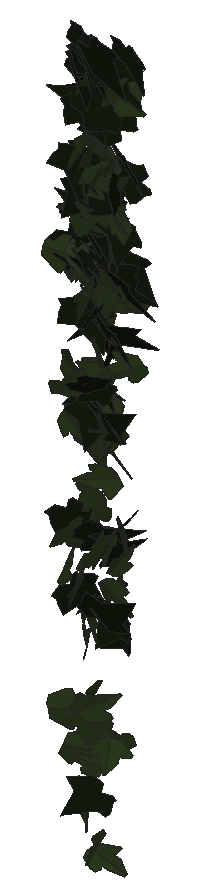
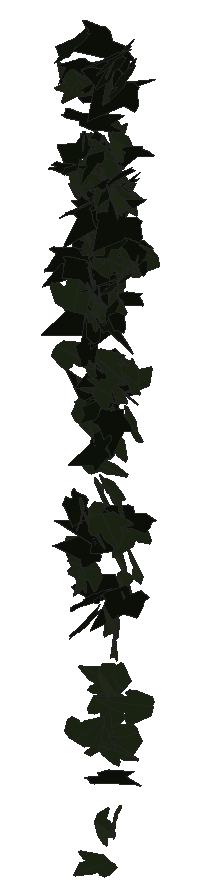
# SketchUp Ruby script. Lengths in inches.
U = 1.inch
M = Sketchup.active_model
def pt(a) = Geom::Point3d.new(a.map { |v| v * U })
def face(e, loops, mat)
  f = e.add_face(loops[0].map { |a| pt(a) })
  loops[1..].each { |l| e.add_face(l.map { |a| pt(a) }).erase! }
  f.material = f.back_material = mat if mat
  f
end
# faces: each face lists its corners as indices into pts; further lists are holes
def faces(e, pts, list, mat = nil) = list.each { |f| face(e, (f[0].is_a?(Array) ? f : [f]).map { |l| l.map { |i| pts[i] } }, mat) }
# xy, xz, yz: faces in a plane at the given z, y or x. An outline is a flat list of corners, or four numbers for a rectangle; further outlines are holes
def ring(l) = l.size == 4 ? [[l[0], l[1]], [l[2], l[1]], [l[2], l[3]], [l[0], l[3]]] : l.each_slice(2).to_a
def flat(e, list, mat, &to3) = list.each { |f| face(e, (f[0].is_a?(Array) ? f : [f]).map { |l| ring(l).map { |u, v| to3.(u, v) } }, mat) }
def xy(e, z, list, mat = nil) = flat(e, list, mat) { |x, y| [x, y, z] }
def xz(e, y, list, mat = nil) = flat(e, list, mat) { |x, z| [x, y, z] }
def yz(e, x, list, mat = nil) = flat(e, list, mat) { |y, z| [x, y, z] }
def lines(e, pts, list) = list.each { |a, b| e.add_line(pt(pts[a]), pt(pts[b])) }
# prism: a flat outline (further loops are holes) pulled along v
def prism(e, loops, v, mat = nil)
  f = face(e, loops, mat); d = Geom::Vector3d.new(v.map { |x| x * U })
  f.pushpull(f.normal.samedirection?(d) ? d.length : -d.length)
end
def box(e, o, s, mat = nil) = prism(e, [[o, [o[0] + s[0], o[1], o[2]], [o[0] + s[0], o[1] + s[1], o[2]], [o[0], o[1] + s[1], o[2]]]], [0, 0, s[2]], mat)
def at(x, y, z, deg = 0) = Geom::Transformation.translation(pt([x, y, z])) * Geom::Transformation.rotation(ORIGIN, Z_AXIS, deg.degrees)
def axes(o, x, y, z) = Geom::Transformation.new([*x, 0, *y, 0, *z, 0, *pt(o).to_a, 1])
def part(name) = M.definitions.add(name)
# library, detail: a bought-in or finely detailed component or shape, given as its bounding box
def library(name, o, s) = part(name).tap { |d| box(d.entities, o, s) }
def detail(e, o, s) = box(e.add_group.entities, o, s)
def put(e, d, t, mat = nil) = e.add_instance(d, t).tap { |i| i.material = mat if mat }
def group(e, t, mat = nil) = e.add_group.tap { |g| g.transformation = t; g.material = mat if mat }.entities
root = M.entities
M.materials.add("1026 AP 7946 SUNNY SIDE UP").color = [254, 231, 186]
M.materials.add("efeu1").color = [18, 25, 13]
M.materials.add("efeu2").color = [43, 57, 29]
c1 = part("ivyleaf_9")
p = [[1.54,2.16,1.25],[1.36,2.04,1.19],[-0.21,0.99,0.68],[-0.71,1.11,0.82],[-0.85,0.86,0.67],[-0.8,0.17,0.21],
  [-0.9,-0.01,0.1],[-0.67,-0.16,-0.02],[-0.08,-0.08,-0.05],[-0.03,-0.6,-0.4],[0.65,-0.88,-0.66],[0.83,-0.6,-0.49],
  [1.29,-0.42,-0.43],[1.8125,-0.07,-0.26],[1.21,0.44,0.15]]
faces(c1.entities,p,[[0,1,2,3,4,5,6,7,8,9,10,11,12,13,14]],"efeu1")
c2 = part("ivyleaf_10")
p = [[0,0.5,-0.03],[-0.0625,2.02,-0.43],[-0.19,2.01,-0.46],[-0.54,1.05,-0.29],[-0.52,0.625,-0.18],[-0.83,0.76,-0.28],
  [-1.16,0.64,-0.33],[-1.15,0.33,-0.24],[-0.77,-0.39,0.02],[-0.3,-0.51,0.16],[0.04,-0.48,0.23],[-0.02,2.01,-0.4375],
  [-0.06,2.01,-0.43],[0.04,-0.49,0.23],[0.67,-0.49,0.14],[1.38,0.36,-0.2],[1.375,0.51,-0.24],[0.81,0.65,-0.19],
  [0.62,0.59,-0.15],[0.6,1.09,-0.28],[0.5,1.23,-0.31]]
faces(c2.entities,p,[[0,1,2,3,4,5,6,7,8,9,10],[11,12,0,13,14,15,16,17,18,19,20]],"efeu2")
put(root,c1,axes([110.53,212.48,267.24],[0.21035,-0.21882,-0.03248],[-0.0439,0.01838,-0.2637],[0.34456,0.13592,-0.01377]),"1026 AP 7946 SUNNY SIDE UP")
put(root,c2,axes([110.8,212.3,263.71],[-0.32704,0.09178,0.06371],[-0.11121,-0.01038,-0.23118],[-0.13325,-0.21659,0.03658]),"1026 AP 7946 SUNNY SIDE UP")
put(root,c2,axes([110.62,212.41,263.32],[-0.07774,0.00799,0.24744],[0.17026,-0.21813,0.02917],[0.33727,0.11196,0.04231]),"1026 AP 7946 SUNNY SIDE UP")
put(root,c2,axes([110.45,212.27,261.32],[0.01134,-0.01111,0.25252],[0.35732,-0.09238,-0.01174],[0.14581,0.22723,0.00913]),"1026 AP 7946 SUNNY SIDE UP")
put(root,c2,axes([110.76,212.29,264.875],[0.02476,-0.20836,0.1301],[-0.00151,-0.12778,-0.21581],[0.38407,0.01293,-0.00924]),"1026 AP 7946 SUNNY SIDE UP")
put(root,c2,axes([110.67,211.92,257.39],[0.2249,-0.21057,0.04235],[-0.014,0.04497,0.26187],[-0.33742,-0.14221,0.01736]),"1026 AP 7946 SUNNY SIDE UP")
put(root,c1,axes([110.58,212.6,263.31],[0.00854,-0.22232,0.09994],[0.03105,-0.09757,-0.22909],[0.38094,0.01294,0.01643]),"1026 AP 7946 SUNNY SIDE UP")
put(root,c2,axes([110.8,212.7,261.2],[-0.02832,-0.12839,0.19332],[-0.04264,-0.18642,-0.13465],[0.35592,-0.03255,-0.00075]),"1026 AP 7946 SUNNY SIDE UP")
put(root,c2,axes([110.41,212.01,263.67],[-0.02831,-0.07099,-0.26298],[0.4153,-0.0198,-0.01365],[-0.0244,-0.25474,0.07273]),"1026 AP 7946 SUNNY SIDE UP")
put(root,c1,axes([110.64,212.21,257.03],[0.03332,-0.08184,-0.27604],[-0.07945,0.26272,-0.0854],[0.43261,0.05455,0.00558]),"1026 AP 7946 SUNNY SIDE UP")
put(root,c2,axes([111.01,212.47,263.63],[-0.10628,-0.027,0.24128],[-0.29259,-0.14375,-0.07319],[0.22802,-0.19705,0.01854]),"1026 AP 7946 SUNNY SIDE UP")
put(root,c1,axes([110.64,212.625,265.39],[0.00168,-0.25128,-0.02336],[0.00658,0.02126,-0.2587],[0.39646,0.00071,0.00439]),"1026 AP 7946 SUNNY SIDE UP")
put(root,c1,axes([110.66,212.32,264.46],[0.32463,0.14976,0.01796],[0.0383,-0.00541,-0.26208],[-0.2338,0.20705,-0.01799]),"1026 AP 7946 SUNNY SIDE UP")
put(root,c1,axes([110.61,212.2,263.97],[-0.00886,-0.04705,-0.2482],[0.08546,0.2345,-0.04717],[0.37599,-0.05441,0.00487]),"1026 AP 7946 SUNNY SIDE UP")
put(root,c2,axes([110.53,212.18,260.33],[0.09967,0.00276,0.24211],[0.34341,-0.0906,-0.06012],[0.13651,0.22591,-0.02554]),"1026 AP 7946 SUNNY SIDE UP")
put(root,c2,axes([110.73,211.93,261.05],[-0.18233,-0.19779,0.08114],[0.05318,0.07273,0.23651],[-0.33117,0.12057,-0.00669]),"1026 AP 7946 SUNNY SIDE UP")
put(root,c2,axes([110.76,212,258.28],[-0.17012,-0.21862,-0.16272],[0.11818,0.13762,-0.25042],[0.4061,-0.13163,0.00471]),"1026 AP 7946 SUNNY SIDE UP")
put(root,c1,axes([110.63,212.1,258.58],[-0.01613,-0.09449,-0.22982],[0.12276,0.20952,-0.09412],[0.3598,-0.07572,0.02181]),"1026 AP 7946 SUNNY SIDE UP")
put(root,c1,axes([110.66,212.55,267.66],[0.03626,-0.25281,0.10174],[0.0069,-0.10019,-0.26207],[0.42754,0.02306,-0.0044]),"1026 AP 7946 SUNNY SIDE UP")
put(root,c2,axes([110.85,212.1,257.2],[0.09037,-0.22921,0.00924],[-0.00391,-0.01121,-0.24345],[0.36075,0.05729,-0.00495]),"1026 AP 7946 SUNNY SIDE UP")
put(root,c2,axes([110.93,212.48,258.51],[-0.23687,-0.16124,0.07836],[-0.06333,-0.06745,-0.22714],[0.27371,-0.15514,0.01526]),"1026 AP 7946 SUNNY SIDE UP")
put(root,c2,axes([110.89,212.4,256.77],[0.04127,-0.23909,-0.00761],[-0.00505,0.00571,-0.24774],[0.37604,0.02631,-0.00249]),"1026 AP 7946 SUNNY SIDE UP")
put(root,c2,axes([110.9,212.41,265.03],[0.13181,-0.23124,-0.04316],[-0.03213,0.03574,-0.25308],[0.36775,0.086,-0.00664]),"1026 AP 7946 SUNNY SIDE UP")
put(root,c2,axes([110.94,212.17,252.58],[0.02923,0.02776,-0.24498],[-0.05835,0.23612,0.02677],[0.37215,0.03484,0.02344]),"1026 AP 7946 SUNNY SIDE UP")
put(root,c1,axes([110.72,212.36,267.11],[0.03723,-0.22168,0.15427],[0.01536,-0.15079,-0.23049],[0.42148,0.02508,-0.00523]),"1026 AP 7946 SUNNY SIDE UP")
put(root,c1,axes([110.75,211.9375,263.59],[0.37651,0.01521,-0.04128],[-0.06017,-0.02762,-0.24602],[-0.03063,0.24122,-0.02413]),"1026 AP 7946 SUNNY SIDE UP")
put(root,c2,axes([110.6,211.9,254.76],[0.051,-0.00885,-0.28812],[0.389,0.13236,0.02602],[0.20542,-0.24844,0.02226]),"1026 AP 7946 SUNNY SIDE UP")
put(root,c2,axes([110.96,212.17,256.04],[0.02352,-0.02907,-0.24498],[-0.05789,0.23498,-0.03063],[0.37196,0.03841,0.01073]),"1026 AP 7946 SUNNY SIDE UP")
put(root,c1,axes([110.72,212.56,263.96],[0.02096,-0.18322,0.1737],[0.0948,-0.16251,-0.18663],[0.38101,0.05051,0.03688]),"1026 AP 7946 SUNNY SIDE UP")
put(root,c1,axes([110.83,212.2,267],[0.2399,0.23699,0.10471],[0.11162,0.07331,-0.28929],[-0.38895,0.16722,-0.01844]),"1026 AP 7946 SUNNY SIDE UP")
put(root,c2,axes([110.93,212.21,267.13],[-0.026,-0.18025,-0.22286],[0.04142,0.21373,-0.18517],[0.43958,-0.0308,0.00427]),"1026 AP 7946 SUNNY SIDE UP")
put(root,c1,axes([110.97,212.28,260.51],[0.27431,0.03959,-0.16722],[-0.24451,-0.04826,-0.18432],[-0.09704,0.23351,-0.00828]),"1026 AP 7946 SUNNY SIDE UP")
put(root,c2,axes([110.89,212.21,265.83],[0.05614,-0.14651,0.20226],[0.07485,-0.19133,-0.15647],[0.37892,0.0595,0.00094]),"1026 AP 7946 SUNNY SIDE UP")
put(root,c1,axes([110.91,212.17,264.85],[-0.10484,-0.16371,0.17331],[-0.0882,-0.1597,-0.18293],[0.35949,-0.08693,0.00566]),"1026 AP 7946 SUNNY SIDE UP")
put(root,c2,axes([110.64,212.09,263.5],[0.05389,-0.03015,0.26577],[0.39459,-0.06394,-0.04239],[0.10638,0.25244,0.0226]),"1026 AP 7946 SUNNY SIDE UP")
put(root,c2,axes([110.91,212.29,256.59],[-0.23412,0.18534,-0.04858],[0.0293,-0.04676,-0.24473],[-0.29969,-0.14936,0.01403]),"1026 AP 7946 SUNNY SIDE UP")
put(root,c1,axes([110.91,212.12,265.6],[-0.19456,-0.22788,-0.06174],[0.06088,0.04563,-0.26658],[0.36494,-0.1291,0.01156]),"1026 AP 7946 SUNNY SIDE UP")
put(root,c2,axes([110.74,212.64,265.71],[-0.1503,0.03877,-0.25334],[0.30139,-0.157,-0.10308],[-0.25034,-0.21229,0.028]),"1026 AP 7946 SUNNY SIDE UP")
put(root,c2,axes([110.93,211.96,263.61],[0.16078,0.07176,-0.21553],[0.09698,0.21253,0.10718],[0.33462,-0.09607,0.0725]),"1026 AP 7946 SUNNY SIDE UP")
put(root,c2,axes([111.25,212.08,253.8],[0.04147,0.05616,0.22779],[-0.35308,-0.03113,0.03561],[0.0605,-0.22017,0.05167]),"1026 AP 7946 SUNNY SIDE UP")
put(root,c2,axes([111.03,212.4,264.85],[-0.05861,-0.22767,0.10131],[0.0141,-0.10192,-0.23706],[0.39052,-0.03049,0.02377]),"1026 AP 7946 SUNNY SIDE UP")
put(root,c1,axes([110.79,212.46,267.34],[0.13987,-0.23061,0.09352],[0.03504,-0.09001,-0.25491],[0.38887,0.09105,-0.01067]),"1026 AP 7946 SUNNY SIDE UP")
put(root,c2,axes([110.84,211.93,254.1],[-0.07548,-0.05933,-0.2541],[0.28105,0.16975,-0.07701],[0.28234,-0.18483,0.00873]),"1026 AP 7946 SUNNY SIDE UP")
put(root,c2,axes([111.08,212.19,259.03],[0.28022,-0.15063,-0.09153],[-0.09917,0.06164,-0.23995],[0.25575,0.18895,0.00724]),"1026 AP 7946 SUNNY SIDE UP")
put(root,c1,axes([111.29,212.28,264.36],[-0.00489,0.05439,0.26295],[-0.40867,0.01897,-0.00733],[-0.03154,-0.25425,0.05414]),"1026 AP 7946 SUNNY SIDE UP")
put(root,c2,axes([111.0625,212.53,262.7],[-0.27687,0.14506,0.01845],[-0.05315,-0.01444,-0.23271],[-0.22343,-0.17632,0.0325]),"1026 AP 7946 SUNNY SIDE UP")
put(root,c1,axes([110.91,212.09,266.74],[0.07886,-0.22501,-0.16973],[-0.0777,0.15626,-0.23627],[0.43037,0.06944,-0.01156]),"1026 AP 7946 SUNNY SIDE UP")
put(root,c2,axes([110.97,212.28,260.03],[-0.37486,0.07125,-0.0784],[0.10308,-0.04651,-0.25534],[-0.12806,-0.24602,0.02395]),"1026 AP 7946 SUNNY SIDE UP")
put(root,c1,axes([110.97,212.53,267.52],[-0.12095,-0.23603,0.08358],[0.00689,-0.08754,-0.25442],[0.39308,-0.07109,0.03018]),"1026 AP 7946 SUNNY SIDE UP")
put(root,c2,axes([111.15,211.96,264.66],[-0.36302,-0.0868,0.06198],[-0.07017,-0.05219,-0.25222],[0.151,-0.23293,0.0318]),"1026 AP 7946 SUNNY SIDE UP")
put(root,c2,axes([111.09,212.01,265.22],[-0.08644,0.22852,0.07859],[-0.09972,0.06042,-0.23724],[-0.36479,-0.07067,0.04623]),"1026 AP 7946 SUNNY SIDE UP")
put(root,c1,axes([111.22,212.34,262.5],[-0.29277,0.18233,-0.08805],[0.07029,-0.07752,-0.26788],[-0.30944,-0.19011,0.02246]),"1026 AP 7946 SUNNY SIDE UP")
put(root,c1,axes([111.14,212.29,264.59],[-0.11265,0.14703,-0.19017],[0.10266,-0.17395,-0.16909],[-0.35767,-0.09624,0.01137]),"1026 AP 7946 SUNNY SIDE UP")
put(root,c2,axes([111.08,212.38,262.87],[0.09055,-0.22927,-0.05622],[0.00382,0.05542,-0.24269],[0.3701,0.05553,0.01626]),"1026 AP 7946 SUNNY SIDE UP")
put(root,c2,axes([111,212.4,263.13],[-0.10245,0.14727,-0.1753],[0.04335,-0.17145,-0.16395],[-0.35219,-0.06394,0.03081]),"1026 AP 7946 SUNNY SIDE UP")
put(root,c2,axes([111.03,212.0625,257.72],[0.17985,-0.19284,0.11996],[0.07845,-0.10692,-0.23136],[0.34633,0.12436,-0.00989]),"1026 AP 7946 SUNNY SIDE UP")
put(root,c1,axes([110.88,212.46,262.58],[0.09867,-0.17785,0.15419],[0.06564,-0.14494,-0.19501],[0.3606,0.07505,-0.00669]),"1026 AP 7946 SUNNY SIDE UP")
put(root,c1,axes([110.93,212.43,264.23],[0.09703,-0.23496,0.00497],[-0.00575,-0.00732,-0.25025],[0.36954,0.06158,-0.0052]),"1026 AP 7946 SUNNY SIDE UP")
put(root,c2,axes([111.26,212.24,261.44],[-0.19776,-0.11935,0.17048],[-0.1582,-0.13375,-0.1782],[0.28009,-0.15981,0.01972]),"1026 AP 7946 SUNNY SIDE UP")
put(root,c2,axes([111.13,212.1,263.07],[0.04487,-0.27898,0.06106],[0.01215,-0.06038,-0.28925],[0.44882,0.02952,0.00173]),"1026 AP 7946 SUNNY SIDE UP")
put(root,c1,axes([111.07,212.48,265.8125],[0.28706,-0.07966,-0.16819],[-0.23347,0.0668,-0.2048],[0.16345,0.23531,0.00284]),"1026 AP 7946 SUNNY SIDE UP")
put(root,c1,axes([111.125,212.49,263.02],[-0.19791,-0.18572,0.09633],[-0.03684,-0.09716,-0.22927],[0.32562,-0.12387,0.03261]),"1026 AP 7946 SUNNY SIDE UP")
put(root,c1,axes([110.9,212.57,259.97],[0.31406,-0.16862,-0.00263],[-0.01843,-0.01142,-0.26883],[0.26451,0.19941,-0.01561]),"1026 AP 7946 SUNNY SIDE UP")
put(root,c2,axes([111.0625,212.65,263.19],[-0.08667,0.16502,-0.18],[0.02694,-0.17706,-0.17792],[-0.37801,-0.05045,0.02859]),"1026 AP 7946 SUNNY SIDE UP")
put(root,c2,axes([110.88,212.18,265.12],[0.30419,-0.11612,-0.16434],[0.24516,-0.04545,0.22956],[-0.18875,-0.24616,0.03333]),"1026 AP 7946 SUNNY SIDE UP")
put(root,c1,axes([110.9,212.49,261.2],[-0.02548,-0.03134,-0.24722],[0.37975,-0.0145,-0.01494],[-0.01963,-0.2399,0.03177]),"1026 AP 7946 SUNNY SIDE UP")
put(root,c2,axes([111.19,212.03,254.68],[-0.29524,-0.18061,0.00847],[0.00951,-0.0196,-0.26784],[0.2842,-0.18697,0.01777]),"1026 AP 7946 SUNNY SIDE UP")
put(root,c2,axes([111.22,212.42,265.28],[-0.22219,-0.20004,0.1054],[-0.02922,-0.11135,-0.24863],[0.35291,-0.13517,0.04577]),"1026 AP 7946 SUNNY SIDE UP")
put(root,c1,axes([111.42,212.49,266.18],[-0.39493,-0.11157,-0.05484],[-0.08425,-0.00879,0.28274],[-0.1747,0.25646,-0.01238]),"1026 AP 7946 SUNNY SIDE UP")
put(root,c1,axes([111.35,212.23,261.25],[-0.38433,0.08216,-0.0109],[0.00451,-0.026,-0.26467],[-0.13027,-0.24329,0.023]),"1026 AP 7946 SUNNY SIDE UP")
put(root,c2,axes([111.22,212.32,264.63],[-0.22236,0.22211,-0.04148],[-0.0194,0.04132,0.27124],[0.35477,0.14147,-0.01116]),"1026 AP 7946 SUNNY SIDE UP")
put(root,c2,axes([111.08,212.47,262.63],[0.18596,-0.21312,0.03412],[-0.00011,0.0391,0.25058],[-0.33942,-0.11677,0.01861]),"1026 AP 7946 SUNNY SIDE UP")
put(root,c1,axes([111.39,212.29,266.64],[-0.15885,-0.24587,-0.14923],[-0.07881,-0.13448,0.27303],[-0.44062,0.1127,0.00497]),"1026 AP 7946 SUNNY SIDE UP")
put(root,c2,axes([111.15,212.34,262.8],[-0.41678,-0.04227,-0.03465],[0.0581,-0.02061,-0.27533],[0.06164,-0.26636,0.0252]),"1026 AP 7946 SUNNY SIDE UP")
put(root,c1,axes([111.02,212.07,262.72],[-0.10397,-0.20496,-0.14951],[0.10395,0.12933,-0.22021],[0.37986,-0.09149,0.01934]),"1026 AP 7946 SUNNY SIDE UP")
put(root,c1,axes([111.09,212.12,262.4375],[0.38117,-0.02202,-0.12216],[-0.18739,-0.00465,-0.25038],[0.02788,0.26977,-0.0127]),"1026 AP 7946 SUNNY SIDE UP")
put(root,c2,axes([111.18,212.3,253.91],[0.0958,0.22313,-0.04432],[0.00883,0.04436,0.23846],[0.35759,-0.06087,0.00599]),"1026 AP 7946 SUNNY SIDE UP")
put(root,c2,axes([111.2,211.97,265.95],[0.08256,-0.25085,-0.09834],[0.00054,0.09588,-0.26276],[0.42124,0.04904,0.01961]),"1026 AP 7946 SUNNY SIDE UP")
put(root,c2,axes([111.18,212.1875,255.25],[0.08259,-0.20416,0.11835],[0.03275,-0.11439,-0.21771],[0.36779,0.05603,-0.00719]),"1026 AP 7946 SUNNY SIDE UP")
put(root,c1,axes([111.3,212.12,253.23],[-0.2796,-0.12947,0.10313],[-0.1098,-0.07487,-0.22631],[0.23353,-0.19022,0.01708]),"1026 AP 7946 SUNNY SIDE UP")
put(root,c1,axes([111.29,212.49,263.43],[0.15602,0.13571,-0.1789],[-0.13746,-0.1515,-0.17355],[-0.31915,0.1316,-0.0127]),"1026 AP 7946 SUNNY SIDE UP")
put(root,c2,axes([111,212.46,251.78],[0.15812,0.1094,0.17871],[0.19047,0.12337,-0.15231],[-0.25921,0.15739,-0.00291]),"1026 AP 7946 SUNNY SIDE UP")
put(root,c1,axes([111.01,211.97,261.25],[0.29906,0.11507,0.10241],[0.15184,0.03024,-0.2277],[-0.18384,0.21216,-0.02146]),"1026 AP 7946 SUNNY SIDE UP")
put(root,c2,axes([111.14,212.51,263.9],[-0.30259,0.10925,-0.08649],[0.08714,-0.07181,-0.22587],[-0.199,-0.19756,0.03261]),"1026 AP 7946 SUNNY SIDE UP")
put(root,c2,axes([111.32,211.9,263.3],[-0.06112,0.10634,0.22772],[-0.18893,0.18617,-0.11325],[-0.33528,-0.12429,0.02231]),"1026 AP 7946 SUNNY SIDE UP")
put(root,c1,axes([111.18,212.15,260.68],[-0.16263,-0.2224,0.0245],[0.00236,-0.02828,-0.25248],[0.3519,-0.10259,0.01302]),"1026 AP 7946 SUNNY SIDE UP")
put(root,c1,axes([111.15,212.43,264.46],[0.0431,-0.09313,-0.26496],[-0.11164,0.24665,-0.09856],[0.41456,0.07611,0.001]),"1026 AP 7946 SUNNY SIDE UP")
put(root,c2,axes([111.44,212.22,259.42],[0.15544,-0.00525,-0.21402],[-0.32334,-0.03548,-0.1001],[-0.04688,0.22729,-0.01921]),"1026 AP 7946 SUNNY SIDE UP")
put(root,c1,axes([110.96,212.39,264.99],[0.27214,-0.24154,0.08439],[0.0496,-0.07963,-0.30589],[0.39867,0.17479,-0.01955]),"1026 AP 7946 SUNNY SIDE UP")
put(root,c1,axes([110.97,212.2,258.06],[0.1039,0.02713,0.27084],[0.39688,0.07336,-0.07277],[-0.12244,0.2608,-0.00605]),"1026 AP 7946 SUNNY SIDE UP")
put(root,c2,axes([111.29,212.18,258.88],[0.20185,-0.20169,-0.04189],[-0.05116,0.02606,-0.24576],[0.31909,0.13177,-0.0129]),"1026 AP 7946 SUNNY SIDE UP")
put(root,c2,axes([111.26,211.91,257.93],[0.13091,-0.1693,0.2181],[-0.10384,0.20316,0.19443],[-0.41462,-0.10433,0.02017]),"1026 AP 7946 SUNNY SIDE UP")
put(root,c1,axes([111.55,212.06,264.96],[-0.16251,0.13238,0.18837],[-0.25355,0.09631,-0.16584],[-0.24705,-0.18592,0.04629]),"1026 AP 7946 SUNNY SIDE UP")
put(root,c2,axes([111.38,212.39,263.45],[0.06174,-0.15029,-0.20047],[-0.10969,0.18125,-0.15835],[0.36962,0.0789,-0.01351]),"1026 AP 7946 SUNNY SIDE UP")
put(root,c1,axes([111.07,212.47,260.66],[0.11264,-0.21484,0.13086],[0.07698,-0.11878,-0.23386],[0.38582,0.08642,0.00846]),"1026 AP 7946 SUNNY SIDE UP")
put(root,c1,axes([111.12,212.13,263.72],[0.18435,-0.20698,-0.08994],[-0.03063,0.08742,-0.24324],[0.35118,0.11628,0.026]),"1026 AP 7946 SUNNY SIDE UP")
put(root,c2,axes([111.41,212.27,260.92],[0.31617,-0.07456,-0.11996],[-0.18621,0.01177,-0.21917],[0.11113,0.23184,-0.02595]),"1026 AP 7946 SUNNY SIDE UP")
put(root,c1,axes([111.39,211.81,262.74],[0.02625,0.15952,0.19413],[0.01496,0.18741,-0.164],[-0.38684,0.01807,0.00683]),"1026 AP 7946 SUNNY SIDE UP")
put(root,c2,axes([111.35,212.05,265.55],[0.06796,-0.23133,-0.13163],[-0.01669,0.12652,-0.24142],[0.41421,0.04305,0.01187]),"1026 AP 7946 SUNNY SIDE UP")
put(root,c2,axes([111.28,212.17,252.3],[0.08689,-0.1524,0.18371],[0.07653,-0.17268,-0.16777],[0.36189,0.07311,-0.00863]),"1026 AP 7946 SUNNY SIDE UP")
put(root,c1,axes([111.04,212.19,267.72],[-0.10604,-0.04605,-0.29578],[0.42507,0.09793,-0.0811],[0.16735,-0.27793,0.01856]),"1026 AP 7946 SUNNY SIDE UP")
put(root,c1,axes([111.27,212.51,261.625],[0.06355,0.14905,0.19582],[-0.12799,-0.17214,0.15658],[0.35649,-0.08837,0.02131]),"1026 AP 7946 SUNNY SIDE UP")
put(root,c2,axes([111.49,212.45,254.1],[-0.25018,-0.07968,-0.14848],[-0.21616,-0.04496,0.18225],[-0.14146,0.20961,-0.01589]),"1026 AP 7946 SUNNY SIDE UP")
put(root,c1,axes([111.19,212.41,264.55],[0.09222,-0.24322,0.00958],[-0.00045,-0.01106,-0.2578],[0.38281,0.05858,-0.00261]),"1026 AP 7946 SUNNY SIDE UP")
put(root,c2,axes([111.22,211.87,254.94],[-0.14992,-0.13926,0.21736],[0.15159,0.18934,0.17408],[-0.3686,0.13451,-0.01682]),"1026 AP 7946 SUNNY SIDE UP")
put(root,c2,axes([111.31,212.125,260.57],[-0.13355,0.20621,-0.13133],[0.0618,-0.12283,-0.23028],[-0.37714,-0.09315,0.00877]),"1026 AP 7946 SUNNY SIDE UP")
put(root,c2,axes([111.32,212.12,265.49],[-0.19327,-0.20674,-0.09385],[0.16351,0.03889,-0.2383],[0.31454,-0.14725,0.06621]),"1026 AP 7946 SUNNY SIDE UP")
put(root,c2,axes([111.31,212.37,258.2],[0.27436,-0.14158,0.10806],[0.10761,-0.08279,-0.23113],[0.25613,0.18645,-0.01864]),"1026 AP 7946 SUNNY SIDE UP")
put(root,c2,axes([111.48,212.62,262.65],[-0.38158,-0.12844,-0.05587],[-0.082,-0.01575,0.28257],[-0.20284,0.248,-0.00914]),"1026 AP 7946 SUNNY SIDE UP")
put(root,c2,axes([111.54,211.81,262.04],[-0.06223,0.11493,-0.20649],[-0.13222,0.18295,0.12584],[0.33934,0.09236,0.01117]),"1026 AP 7946 SUNNY SIDE UP")
put(root,c2,axes([111.55,212.24,260.18],[-0.16025,-0.09379,-0.20834],[-0.20281,-0.15584,0.14088],[-0.28497,0.16366,0.01689]),"1026 AP 7946 SUNNY SIDE UP")
put(root,c1,axes([111.29,212.32,257.78],[0.07184,0.05556,0.24422],[0.27613,0.1591,-0.07245],[-0.26451,0.18118,-0.0093]),"1026 AP 7946 SUNNY SIDE UP")
put(root,c1,axes([111.39,212.58,256.28],[-0.11433,-0.13801,0.22519],[-0.05846,-0.21993,-0.15652],[0.40331,-0.071,0.04115]),"1026 AP 7946 SUNNY SIDE UP")
put(root,c2,axes([111.46,212.29,265.64],[0.03477,-0.24488,-0.03933],[0.01628,0.03781,-0.25269],[0.38902,0.0203,0.01409]),"1026 AP 7946 SUNNY SIDE UP")
put(root,c1,axes([111.27,212.51,267.35],[-0.02196,-0.20404,-0.16654],[0.09994,0.15315,-0.20538],[0.39576,-0.05,0.04262]),"1026 AP 7946 SUNNY SIDE UP")
put(root,c2,axes([111.51,212.14,260.14],[0.08349,-0.21373,-0.06173],[-0.02216,0.05699,-0.22655],[0.34782,0.05493,0.00038]),"1026 AP 7946 SUNNY SIDE UP")
put(root,c2,axes([111.34,212.3125,264.79],[-0.2533,0.0827,-0.17423],[0.17522,-0.13824,-0.1793],[-0.23941,-0.18868,0.0531]),"1026 AP 7946 SUNNY SIDE UP")
put(root,c2,axes([111.49,212.07,258.26],[0.03587,-0.21802,0.10898],[0.02918,-0.10562,-0.22634],[0.38078,0.02863,0.00708]),"1026 AP 7946 SUNNY SIDE UP")
put(root,c2,axes([111.38,212.39,263.92],[0.03286,-0.13643,-0.24719],[0.06056,-0.23605,0.1408],[-0.42869,-0.04381,0.00094]),"1026 AP 7946 SUNNY SIDE UP")
put(root,c2,axes([111.53,212.51,265.16],[0.01459,-0.25034,0.05187],[0.00348,-0.05173,-0.25838],[0.40196,0.00953,0.00035]),"1026 AP 7946 SUNNY SIDE UP")
put(root,c2,axes([111.55,212.34,257.21],[0.01503,-0.09076,-0.23238],[-0.01268,0.22499,-0.09251],[0.38137,0.01105,0.00608]),"1026 AP 7946 SUNNY SIDE UP")
put(root,c2,axes([111.48,212.17,254.2],[0.20599,0.19269,-0.06107],[-0.04087,-0.05527,-0.24017],[-0.31487,0.13323,-0.00877]),"1026 AP 7946 SUNNY SIDE UP")
put(root,c2,axes([111.58,212.12,263.18],[-0.2456,-0.20709,0.02798],[-0.00763,-0.03177,-0.26695],[0.32857,-0.15553,0.01472]),"1026 AP 7946 SUNNY SIDE UP")
put(root,c1,axes([111.77,212.61,265.18],[-0.30789,-0.00854,0.14556],[-0.21053,-0.06733,-0.19567],[0.07246,-0.23192,0.04998]),"1026 AP 7946 SUNNY SIDE UP")
put(root,c2,axes([111.68,212.18,264.59],[0.26778,-0.08911,-0.15941],[-0.23674,0.04202,-0.19603],[0.14968,0.22589,-0.02485]),"1026 AP 7946 SUNNY SIDE UP")
put(root,c1,axes([111.53,212.3125,256.65],[-0.14299,-0.18845,0.12696],[-0.06956,-0.11654,-0.21603],[0.3481,-0.1007,0.00898]),"1026 AP 7946 SUNNY SIDE UP")
put(root,c1,axes([111.3125,212.11,260.41],[-0.09709,0.03762,0.24317],[0.30043,-0.13835,0.07346],[0.22528,0.20072,0.00684]),"1026 AP 7946 SUNNY SIDE UP")
put(root,c2,axes([111.48,212.42,267],[-0.13356,-0.19063,-0.16536],[0.14564,0.13206,-0.21274],[0.3626,-0.12326,0.02454]),"1026 AP 7946 SUNNY SIDE UP")
put(root,c2,axes([111.73,212.55,261.58],[-0.1615,-0.06527,0.21544],[-0.19724,-0.17232,-0.11967],[0.28308,-0.1573,0.03953]),"1026 AP 7946 SUNNY SIDE UP")
put(root,c2,axes([111.5,212.33,257.62],[0.01124,-0.18976,0.15034],[-0.01078,0.14686,0.19649],[-0.3773,-0.00985,-0.00114]),"1026 AP 7946 SUNNY SIDE UP")
put(root,c2,axes([111.77,211.82,263.43],[0.08961,-0.06956,-0.26098],[-0.25988,0.19149,-0.09149],[0.32033,0.17481,-0.00122]),"1026 AP 7946 SUNNY SIDE UP")
put(root,c1,axes([111.69,212.39,258.58],[-0.18493,0.16326,-0.14179],[0.10307,-0.12305,-0.20739],[-0.32054,-0.13376,0.01511]),"1026 AP 7946 SUNNY SIDE UP")
put(root,c1,axes([111.39,212.14,262.48],[0.25844,-0.20785,0.00003],[-0.0194,-0.01129,-0.27251],[0.32625,0.16398,-0.01622]),"1026 AP 7946 SUNNY SIDE UP")
put(root,c1,axes([111.39,212.25,262.22],[0.31681,0.10798,0.13292],[0.18868,0.04752,-0.23484],[-0.18439,0.23415,-0.01192]),"1026 AP 7946 SUNNY SIDE UP")
put(root,c1,axes([111.39,212.03,256.74],[-0.10858,0.00326,0.25043],[0.32266,-0.13469,0.06113],[0.20492,0.2138,0.03644]),"1026 AP 7946 SUNNY SIDE UP")
put(root,c1,axes([111.38,212.65,265.52],[0.13941,-0.19704,0.16099],[0.0735,-0.1511,-0.22289],[0.38966,0.099,-0.01555]),"1026 AP 7946 SUNNY SIDE UP")
put(root,c1,axes([111.81,211.94,265.375],[0.03891,-0.04185,-0.26962],[-0.39884,0.07167,-0.03613],[0.11958,0.25268,-0.03277]),"1026 AP 7946 SUNNY SIDE UP")
put(root,c1,axes([111.46,212.23,263.375],[0.05755,-0.07652,-0.2881],[-0.01446,0.281,-0.07893],[0.45501,0.01861,0.03393]),"1026 AP 7946 SUNNY SIDE UP")
put(root,c1,axes([111.42,212.54,263.55],[-0.05657,-0.12553,-0.2183],[0.19323,0.17563,-0.12808],[0.33451,-0.12268,0.03707]),"1026 AP 7946 SUNNY SIDE UP")
put(root,c2,axes([111.45,212.22,257.28],[-0.22794,0.06971,-0.1843],[0.23572,-0.09975,-0.1654],[-0.18956,-0.20787,0.01593]),"1026 AP 7946 SUNNY SIDE UP")
put(root,c2,axes([111.57,212.37,258.45],[-0.17586,0.19834,-0.08859],[0.0531,-0.08088,-0.23484],[-0.33647,-0.11643,0.00924]),"1026 AP 7946 SUNNY SIDE UP")
put(root,c2,axes([111.42,212.4,266.75],[0.34325,0.02044,-0.16372],[0.24288,0.04526,0.22469],[0.06763,-0.26627,0.02401]),"1026 AP 7946 SUNNY SIDE UP")
put(root,c1,axes([111.36,212.22,263.37],[0.41429,-0.10234,0.07204],[0.08434,-0.05545,-0.28972],[0.17627,0.26705,-0.03069]),"1026 AP 7946 SUNNY SIDE UP")
put(root,c1,axes([111.59,212.37,264.36],[-0.08332,-0.23729,0.06041],[-0.00148,-0.06118,-0.25052],[0.38484,-0.05161,0.01212]),"1026 AP 7946 SUNNY SIDE UP")
put(root,c1,axes([111.48,212.64,267.66],[0.10729,-0.24135,0.07467],[0.03639,-0.0702,-0.25877],[0.39519,0.07199,0.00356]),"1026 AP 7946 SUNNY SIDE UP")
